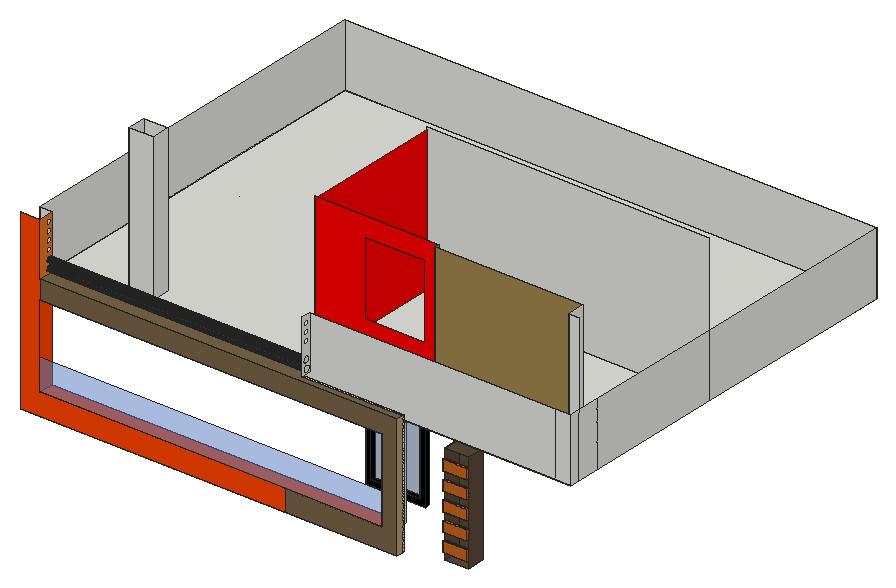
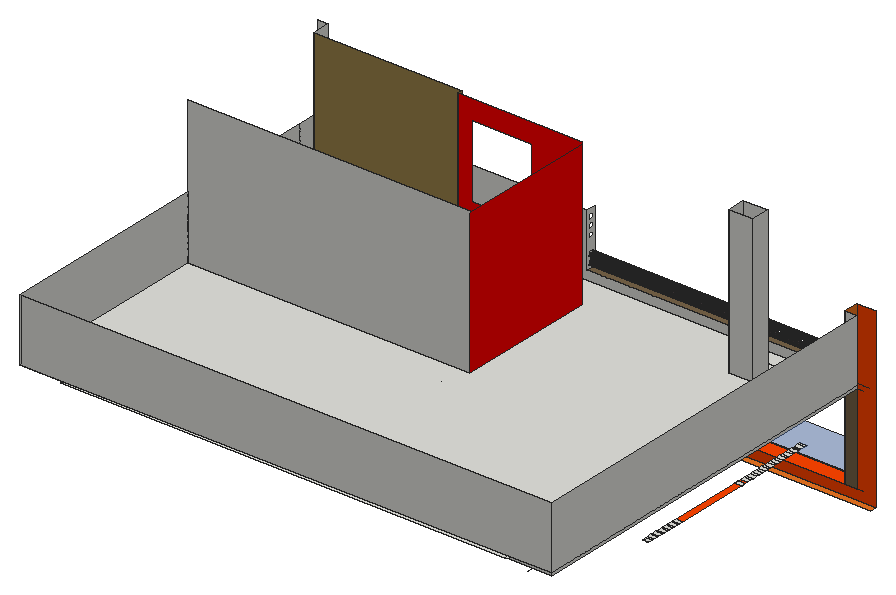
# SketchUp Ruby script. Lengths in inches.
U = 1.inch
M = Sketchup.active_model
def pt(a) = Geom::Point3d.new(a.map { |v| v * U })
def face(e, loops, mat)
  f = e.add_face(loops[0].map { |a| pt(a) })
  loops[1..].each { |l| e.add_face(l.map { |a| pt(a) }).erase! }
  f.material = f.back_material = mat if mat
  f
end
# faces: each face lists its corners as indices into pts; further lists are holes
def faces(e, pts, list, mat = nil) = list.each { |f| face(e, (f[0].is_a?(Array) ? f : [f]).map { |l| l.map { |i| pts[i] } }, mat) }
# xy, xz, yz: faces in a plane at the given z, y or x. An outline is a flat list of corners, or four numbers for a rectangle; further outlines are holes
def ring(l) = l.size == 4 ? [[l[0], l[1]], [l[2], l[1]], [l[2], l[3]], [l[0], l[3]]] : l.each_slice(2).to_a
def flat(e, list, mat, &to3) = list.each { |f| face(e, (f[0].is_a?(Array) ? f : [f]).map { |l| ring(l).map { |u, v| to3.(u, v) } }, mat) }
def xy(e, z, list, mat = nil) = flat(e, list, mat) { |x, y| [x, y, z] }
def xz(e, y, list, mat = nil) = flat(e, list, mat) { |x, z| [x, y, z] }
def yz(e, x, list, mat = nil) = flat(e, list, mat) { |y, z| [x, y, z] }
def lines(e, pts, list) = list.each { |a, b| e.add_line(pt(pts[a]), pt(pts[b])) }
# prism: a flat outline (further loops are holes) pulled along v
def prism(e, loops, v, mat = nil)
  f = face(e, loops, mat); d = Geom::Vector3d.new(v.map { |x| x * U })
  f.pushpull(f.normal.samedirection?(d) ? d.length : -d.length)
end
def box(e, o, s, mat = nil) = prism(e, [[o, [o[0] + s[0], o[1], o[2]], [o[0] + s[0], o[1] + s[1], o[2]], [o[0], o[1] + s[1], o[2]]]], [0, 0, s[2]], mat)
def at(x, y, z, deg = 0) = Geom::Transformation.translation(pt([x, y, z])) * Geom::Transformation.rotation(ORIGIN, Z_AXIS, deg.degrees)
def axes(o, x, y, z) = Geom::Transformation.new([*x, 0, *y, 0, *z, 0, *pt(o).to_a, 1])
def part(name) = M.definitions.add(name)
# library, detail: a bought-in or finely detailed component or shape, given as its bounding box
def library(name, o, s) = part(name).tap { |d| box(d.entities, o, s) }
def detail(e, o, s) = box(e.add_group.entities, o, s)
def put(e, d, t, mat = nil) = e.add_instance(d, t).tap { |i| i.material = mat if mat }
def group(e, t, mat = nil) = e.add_group.tap { |g| g.transformation = t; g.material = mat if mat }.entities
root = M.entities
M.materials.add("[0020_Red]").color = [255, 0, 0]
M.materials.add("[0024_OrangeRed]").color = [255, 69, 0]
M.materials.add("[0036_BurlyWood]1").color = [119, 99, 72]
M.materials.add("[0036_BurlyWood]2").color = [181, 150, 110]
M.materials.add("[0036_BurlyWood]3").color = [89, 73, 54]
M.materials.add("[0036_BurlyWood]5").color = [122, 101, 74]
M.materials.add("[0041_Chocolate]").color = [234, 117, 33]
M.materials.add("[0041_Chocolate]2").color = [198, 99, 28]
M.materials.add("[0137_Black]").color = [0, 0, 0]
M.materials.add("[Asphalt New]").color = [67, 60, 62]
M.materials.add("[Brick Rough Tan]").color = [158, 133, 77]
M.materials.add("[Translucent Glass Blue]").color = [51, 76, 122]
M.materials["[Translucent Glass Blue]"].alpha = 0.5
M.materials.add("[Translucent Glass Blue]1").color = [100, 149, 237]
M.materials["[Translucent Glass Blue]1"].alpha = 0.5
M.materials.add("[Wood Floor]").color = [155, 105, 61]
xy(root,214.625,[[0,236.25,504.125,245.125]],"[0041_Chocolate]")
xy(root,226.86,[[561.28,245.125,593.09,268.0625]],"[0036_BurlyWood]3")
xy(root,228.95,[[398.32,315.9375,478.64,321.9375]],"[0137_Black]")
xy(root,235.22,[[230.26,515.4375,307.58,521.4375]],"[0137_Black]")
xy(root,236.21,[[405.59,315.9375,438.48,321.9375],[447.89,315.9375,471.37,321.9375]],"[0137_Black]")
xy(root,236.74,[[561.28,242.125,593.09,245.125]],"[0041_Chocolate]2")
xy(root,241.22,[[236.26,515.4375,268.92,521.4375],[275.71,515.4375,301.58,521.4375]],"[0137_Black]")
xy(root,243,[[25.71,236.25,484.29,257.25]],"[0024_OrangeRed]")
xy(root,250.24,[[561.28,242.125,593.09,245.125]],"[0041_Chocolate]2")
xy(root,261.24,[[561.28,242.125,593.09,245.125]],"[0041_Chocolate]2")
xy(root,274.74,[[561.28,242.125,593.09,245.125]],"[0041_Chocolate]2")
xy(root,285.74,[[561.28,242.125,593.09,245.125]],"[0041_Chocolate]2")
xy(root,299.24,[[561.28,242.125,593.09,245.125]],"[0041_Chocolate]2")
xy(root,310.24,[[561.28,242.125,593.09,245.125]],"[0041_Chocolate]2")
xy(root,317.78,[[236.26,515.4375,268.92,521.4375],[275.71,515.4375,301.58,521.4375]],"[0137_Black]")
xy(root,323.74,[[561.28,242.125,593.09,245.125]],"[0041_Chocolate]2")
xy(root,323.78,[[230.26,515.4375,307.58,521.4375]],"[0137_Black]")
xy(root,326.0625,[[109.24,515.4375,148.77,521.4375],[155.35,515.4375,188.31,521.4375]],"[0137_Black]")
xy(root,330.81,[[405.59,315.9375,438.48,321.9375],[447.89,315.9375,471.37,321.9375]],"[0137_Black]")
xy(root,334.375,[[348.4375,372.41,351.4375,446.78]])
xy(root,334.74,[[561.28,242.125,593.09,245.125]],"[0041_Chocolate]2")
xy(root,335.17,[[100.13,515.4375,197.41,521.4375]])
xy(root,338.07,[[398.32,315.9375,478.64,321.9375]],"[0137_Black]")
xy(root,339.56,[[0,352.64,9,355.7],[0,355.7,9,361.9],[0,361.9,9,365.65],[0,365.65,9,365.7],[0,365.7,9,371.9],
  [0,371.9,9,375.7],[0,375.7,9,381.9],[0,381.9,9,385.7],[0,385.7,9,391.9],[0,391.9,9,395.7],
  [0,395.7,9,401.9],[0,401.9,9,405.7],[0,405.7,9,411.9],[0,411.9,9,415.7],[0,415.7,9,421.9],
  [0,421.9,9,425.7],[0,425.7,9,431.9],[0,431.9,9,435.7],[0,435.7,9,441.9],[0,441.9,9,445.7],
  [0,445.7,9,451.9],[0,559.26,9,565.46],[0,565.46,9,567.7],[0,567.7,9,573.9],[0,573.9,9,576.14],
  [0,576.14,9,582.34],[0,582.34,9,584.57],[0,584.57,9,590.78],[0,590.78,9,593.01],[0,593.01,9,599.21],
  [0,599.21,9,601.45],[0,601.45,9,607.65],[0,607.65,9,609.89],[0,609.89,9,616.09],[0,616.09,9,616.14]])
xy(root,339.56,[[0,451.9,9,559.26]],"[0024_OrangeRed]")
xy(root,339.69,[[0,455.7,9,461.9]])
xy(root,345.77,[[348.4375,361.01,354.4375,458.18]],"[Wood Floor]")
xy(root,348.24,[[561.28,242.125,593.09,245.125]],"[0041_Chocolate]2")
xy(root,354.29,[[25.71,236.25,484.29,257.25]],"[0036_BurlyWood]1")
xy(root,360.8,[[561.28,245.125,593.09,268.0625]],"[0036_BurlyWood]3")
xy(root,363,[[354.4375,321.9375,354.4375,521.4375,360.4375,521.4375,360.4375,327.9375,665.75,327.9375,665.75,321.9375],[665.75,321.9375,698.375,521.4375],[360.4375,327.9375,665.75,521.4375],[65.25,521.4375,354.4375,527.4375],[354.4375,521.4375,360.4375,527.4375],
  [360.4375,521.4375,665.75,527.4375],[65.25,527.4375,71.25,767.8125],[71.25,527.4375,665.75,767.8125]])
xy(root,363,[[9,257.25,9,767.8125,65.25,767.8125,65.25,521.4375,354.4375,521.4375,354.4375,321.9375,498.8125,321.9375,498.8125,257.25]],"[0036_BurlyWood]5")
xy(root,366,[[[9,257.25,720.125,257.25,720.125,270.98,706.26,270.98,706.26,294.98,507.58,294.98,507.58,300.98,342.3125,300.98,342.3125,488.35,720.125,488.35,720.125,767.8125,9,767.8125],[99.47,277.08,132.15,318.33]],[706.26,270.98,720.125,270.98,720.125,300.98,507.58,300.98,507.58,294.98,706.26,294.98],[99.47,277.08,132.15,293.9],[99.47,293.9,132.15,297.46],[99.47,297.46,132.15,318.33],
  [342.3125,300.98,720.125,488.35]])
xy(root,378.625,[[369.99,245.125,504.125,248.25]])
xy(root,378.625,[[25.71,236.25,504.125,236.25,504.125,245.125,369.99,245.125,369.99,257.25,25.71,257.25]],"[0036_BurlyWood]1")
xz(root,236.25,[[0,214.625,353.27,214.625,353.27,243,25.71,243,25.71,450,0,450]],"[0024_OrangeRed]")
xz(root,236.25,[[353.27,214.625,504.125,214.625,504.125,378.625,25.71,378.625,25.71,354.29,484.29,354.29,484.29,243,353.27,243]],"[0036_BurlyWood]1")
xz(root,236.25,[[25.71,243,484.29,285.4]],"[Translucent Glass Blue]1")
xz(root,242.125,[[561.28,236.74,593.09,250.24],[561.28,261.24,593.09,274.74],[561.28,285.74,593.09,299.24],[561.28,310.24,593.09,323.74],[561.28,334.74,593.09,348.24]],"[0041_Chocolate]2")
xz(root,245.125,[[561.28,236.74,593.09,250.24],[561.28,261.24,593.09,274.74],[561.28,285.74,593.09,299.24],[561.28,310.24,593.09,323.74],[561.28,334.74,593.09,348.24]])
xz(root,248.25,[[498.8125,243,504.125,363]])
xz(root,257.25,[[9,366,9,450,25.71,450,25.71,378.625,369.99,378.625,369.99,450,698.375,450,698.375,366],[698.375,366,720.125,450]])
xz(root,257.25,[[9,243,9,363,498.8125,363,498.8125,243,484.29,243,484.29,354.29,25.71,354.29,25.71,243]],"[0036_BurlyWood]1")
xz(root,268.0625,[[561.28,226.86,593.09,360.8]],"[0036_BurlyWood]3")
xz(root,270.98,[[706.26,366,720.125,561.0625]])
xz(root,293.9,[[99.47,366,132.15,561.0625]])
xz(root,294.98,[[507.58,366,706.26,561.0625]],"[Brick Rough Tan]")
xz(root,300.98,[[[342.3125,366,507.58,561.0625],[408.85,437.16,489.23,535.66]]],"[0020_Red]")
xz(root,315.9375,[[[398.32,228.95,478.64,338.07],[405.59,236.21,438.48,330.81],[447.89,236.21,471.37,330.81]]],"[0137_Black]")
xz(root,318.33,[[99.47,366,132.15,561.0625]])
xz(root,321.9375,[[405.59,236.21,438.48,330.81],[447.89,236.21,471.37,330.81]],"[Translucent Glass Blue]")
xz(root,488.35,[[342.3125,366,720.125,561.0625]])
xz(root,515.4375,[[[230.26,235.22,307.58,323.78],[236.26,241.22,268.92,317.78],[275.71,241.22,301.58,317.78]]],"[0137_Black]")
xz(root,521.4375,[[236.26,241.22,268.92,317.78],[275.71,241.22,301.58,317.78]],"[Translucent Glass Blue]")
xz(root,767.8125,[[9,363,65.25,366],[9,366,720.125,450]])
yz(root,0,[[455.7,339.56,461.9,339.69]])
yz(root,9,[[455.7,339.56,461.9,339.69],[257.25,363,767.8125,366],[257.25,366,767.8125,450]])
yz(root,25.71,[[236.25,243,257.25,354.29]],"[0024_OrangeRed]")
yz(root,25.71,[[[236.25,378.625,257.25,450],[251.48,382.01,250.54,382.14,249.67,382.5,248.92,383.07,248.34,383.82,247.98,384.7,247.86,385.64,247.98,386.58,248.34,387.45,248.92,388.2,249.67,388.78,250.54,389.14,251.48,389.26,252.42,389.14,253.3,388.78,254.05,388.2,254.62,387.45,254.98,386.58,255.11,385.64,254.98,384.7,254.62,383.82,254.05,383.07,253.3,382.5,252.42,382.14],[251.48,392.95,250.54,393.07,249.67,393.44,248.92,394.01,248.34,394.76,247.98,395.64,247.86,396.57,247.98,397.51,248.34,398.39,248.92,399.14,249.67,399.71,250.54,400.08,251.48,400.2,252.42,400.08,253.3,399.71,254.05,399.14,254.62,398.39,254.98,397.51,255.11,396.57,254.98,395.64,254.62,394.76,254.05,394.01,253.3,393.44,252.42,393.07],[251.48,403.89,250.54,404.01,249.67,404.37,248.92,404.95,248.34,405.7,247.98,406.57,247.86,407.51,247.98,408.45,248.34,409.32,248.92,410.08,249.67,410.65,250.54,411.01,251.48,411.14,252.42,411.01,253.3,410.65,254.05,410.08,254.62,409.32,254.98,408.45,255.11,407.51,254.98,406.57,254.62,405.7,254.05,404.95,253.3,404.37,252.42,404.01],[251.48,414.82,250.54,414.95,249.67,415.31,248.92,415.89,248.34,416.64,247.98,417.51,247.86,418.45,247.98,419.39,248.34,420.26,248.92,421.01,249.67,421.59,250.54,421.95,251.48,422.07,252.42,421.95,253.3,421.59,254.05,421.01,254.62,420.26,254.98,419.39,255.11,418.45,254.98,417.51,254.62,416.64,254.05,415.89,253.3,415.31,252.42,414.95],[251.48,425.76,250.54,425.89,249.67,426.25,248.92,426.82,248.34,427.57,247.98,428.45,247.86,429.39,247.98,430.33,248.34,431.2,248.92,431.95,249.67,432.53,250.54,432.89,251.48,433.01,252.42,432.89,253.3,432.53,254.05,431.95,254.62,431.2,254.98,430.33,255.11,429.39,254.98,428.45,254.62,427.57,254.05,426.82,253.3,426.25,252.42,425.89],[251.48,436.7,250.54,436.82,249.67,437.19,248.92,437.76,248.34,438.51,247.98,439.39,247.86,440.32,247.98,441.26,248.34,442.14,248.92,442.89,249.67,443.46,250.54,443.83,251.48,443.95,252.42,443.83,253.3,443.46,254.05,442.89,254.62,442.14,254.98,441.26,255.11,440.32,254.98,439.39,254.62,438.51,254.05,437.76,253.3,437.19,252.42,436.82]]],"[0041_Chocolate]")
yz(root,99.47,[[293.9,366,318.33,561.0625]])
yz(root,132.15,[[293.9,366,318.33,561.0625]])
yz(root,230.26,[[515.4375,235.22,521.4375,323.78]],"[0137_Black]")
yz(root,236.26,[[515.4375,241.22,521.4375,317.78]],"[0137_Black]")
yz(root,268.92,[[515.4375,241.22,521.4375,317.78]],"[0137_Black]")
yz(root,275.71,[[515.4375,241.22,521.4375,317.78]],"[0137_Black]")
yz(root,301.58,[[515.4375,241.22,521.4375,317.78]],"[0137_Black]")
yz(root,307.58,[[515.4375,235.22,521.4375,323.78]],"[0137_Black]")
yz(root,342.3125,[[300.98,366,488.35,557.75]],"[0020_Red]")
yz(root,348.4375,[[427.62,258.41,424.34,258.68,421.23,259.79,418.52,261.66,416.39,264.17,414.98,267.15,414.39,270.4,414.66,273.68,415.76,276.78,417.64,279.49,420.15,281.63,423.13,283.04,426.37,283.63,429.66,283.36,432.76,282.25,435.47,280.38,437.6,277.87,439.02,274.89,439.61,271.65,439.34,268.36,438.23,265.26,436.36,262.55,433.84,260.41,430.86,259]],"[Wood Floor]")
yz(root,369.99,[[[245.125,378.625,257.25,450],[251.48,392.95,252.42,393.07,253.3,393.44,254.05,394.01,254.62,394.76,254.98,395.64,255.11,396.57,254.98,397.51,254.62,398.39,254.05,399.14,253.3,399.71,252.42,400.08,251.48,400.2,250.54,400.08,249.67,399.71,248.92,399.14,248.34,398.39,248.25,398.16,247.98,397.51,247.86,396.57,247.98,395.64,248.25,394.99,248.34,394.76,248.92,394.01,249.67,393.44,250.54,393.07],[251.48,414.82,252.42,414.95,253.3,415.31,254.05,415.89,254.62,416.64,254.98,417.51,255.11,418.45,254.98,419.39,254.62,420.26,254.05,421.01,253.3,421.59,252.42,421.95,251.48,422.07,250.54,421.95,249.67,421.59,248.92,421.01,248.34,420.26,248.25,420.04,247.98,419.39,247.86,418.45,247.98,417.51,248.25,416.86,248.34,416.64,248.92,415.89,249.67,415.31,250.54,414.95],[251.48,436.7,252.42,436.82,253.3,437.19,254.05,437.76,254.62,438.51,254.98,439.39,255.11,440.32,254.98,441.26,254.62,442.14,254.05,442.89,253.3,443.46,252.42,443.83,251.48,443.95,250.54,443.83,249.67,443.46,248.92,442.89,248.34,442.14,248.25,441.91,247.98,441.26,247.86,440.32,247.98,439.39,248.25,438.74,248.34,438.51,248.92,437.76,249.67,437.19,250.54,436.82],[251.48,425.76,252.42,425.89,253.3,426.25,254.05,426.82,254.62,427.57,254.98,428.45,255.11,429.39,254.98,430.33,254.62,431.2,254.05,431.95,253.3,432.53,252.42,432.89,251.48,433.01,250.54,432.89,249.67,432.53,248.92,431.95,248.34,431.2,248.25,430.97,247.98,430.33,247.86,429.39,247.98,428.45,248.25,427.8,248.34,427.57,248.92,426.82,249.67,426.25,250.54,425.89]],[251.48,392.95,252.42,393.07,253.3,393.44,254.05,394.01,254.62,394.76,254.98,395.64,255.11,396.57,254.98,397.51,254.62,398.39,254.05,399.14,253.3,399.71,252.42,400.08,251.48,400.2,250.54,400.08,249.67,399.71,248.92,399.14,248.34,398.39,248.25,398.16,248.25,394.99,248.34,394.76,248.92,394.01,249.67,393.44,250.54,393.07],[248.25,394.99,247.98,395.64,247.86,396.57,247.98,397.51,248.25,398.16]])
yz(root,371.08,[[251.48,382.01,252.42,382.14,253.3,382.5,254.05,383.07,254.62,383.82,254.98,384.7,255.11,385.64,254.98,386.58,254.62,387.45,254.05,388.2,253.3,388.78,252.42,389.14,251.48,389.26,250.54,389.14,249.67,388.78,248.92,388.2,248.34,387.45,247.98,386.58,247.86,385.64,247.98,384.7,248.34,383.82,248.92,383.07,249.67,382.5,250.54,382.14]])
yz(root,398.32,[[315.9375,228.95,321.9375,338.07]],"[0137_Black]")
yz(root,405.59,[[315.9375,236.21,321.9375,330.81]],"[0137_Black]")
yz(root,438.48,[[315.9375,236.21,321.9375,330.81]],"[0137_Black]")
yz(root,447.89,[[315.9375,236.21,321.9375,330.81]],"[0137_Black]")
yz(root,471.37,[[315.9375,236.21,321.9375,330.81]],"[0137_Black]")
yz(root,478.64,[[315.9375,228.95,321.9375,338.07]],"[0137_Black]")
yz(root,484.29,[[236.25,243,257.25,354.29]],"[0036_BurlyWood]1")
yz(root,498.8125,[[248.25,243,257.25,363]])
yz(root,504.125,[[245.125,214.625,248.25,243],[245.125,243,248.25,363],[245.125,363,248.25,378.625]])
yz(root,504.125,[[236.25,214.625,245.125,378.625]],"[0036_BurlyWood]2")
yz(root,507.58,[[294.98,366,300.98,561.0625]],"[Brick Rough Tan]")
yz(root,561.28,[[245.125,226.86,268.0625,360.8]],"[0036_BurlyWood]3")
yz(root,561.28,[[242.125,236.74,245.125,250.24],[242.125,261.24,245.125,274.74],[242.125,285.74,245.125,299.24],[242.125,310.24,245.125,323.74],[242.125,334.74,245.125,348.24]],"[0041_Chocolate]2")
yz(root,593.09,[[245.125,226.86,268.0625,360.8]],"[0036_BurlyWood]3")
yz(root,593.09,[[242.125,236.74,245.125,250.24],[242.125,261.24,245.125,274.74],[242.125,285.74,245.125,299.24],[242.125,310.24,245.125,323.74],[242.125,334.74,245.125,348.24]],"[0041_Chocolate]2")
yz(root,706.26,[[270.98,366,294.98,561.0625]])
yz(root,720.125,[[257.25,366,270.98,450],[270.98,366,300.98,450],[300.98,366,488.35,450],[488.35,366,767.8125,450]])
p = [[351.4375,427.62,258.41],[351.4375,424.34,258.68],[348.4375,424.34,258.68],[348.4375,427.62,258.41],[351.4375,430.86,259],[348.4375,430.86,259],
  [351.4375,421.23,259.79],[348.4375,421.23,259.79],[351.4375,433.84,260.41],[348.4375,433.84,260.41],[351.4375,418.52,261.66],[348.4375,418.52,261.66],
  [351.4375,436.36,262.55],[348.4375,436.36,262.55],[351.4375,416.39,264.17],[348.4375,416.39,264.17],[351.4375,438.23,265.26],[348.4375,438.23,265.26],
  [351.4375,414.98,267.15],[348.4375,414.98,267.15],[351.4375,439.34,268.36],[348.4375,439.34,268.36],[351.4375,414.39,270.4],[348.4375,414.39,270.4],
  [351.4375,439.61,271.65],[348.4375,439.61,271.65],[351.4375,414.66,273.68],[348.4375,414.66,273.68],[351.4375,439.02,274.89],[348.4375,439.02,274.89],
  [351.4375,415.76,276.78],[348.4375,415.76,276.78],[351.4375,437.6,277.87],[348.4375,437.6,277.87],[351.4375,417.64,279.49],[348.4375,417.64,279.49],
  [351.4375,435.47,280.38],[348.4375,435.47,280.38],[351.4375,420.15,281.63],[348.4375,420.15,281.63],[351.4375,432.76,282.25],[348.4375,432.76,282.25],
  [351.4375,423.13,283.04],[348.4375,423.13,283.04],[351.4375,429.66,283.36],[348.4375,429.66,283.36],[351.4375,426.37,283.63],[348.4375,426.37,283.63],
  [25.71,250.54,382.14],[25.71,251.48,382.01],[371.08,251.48,382.01],[371.08,250.54,382.14],[25.71,252.42,382.14],[371.08,252.42,382.14],
  [25.71,249.67,382.5],[371.08,249.67,382.5],[25.71,253.3,382.5],[371.08,253.3,382.5],[25.71,248.92,383.07],[371.08,248.92,383.07],
  [25.71,254.05,383.07],[371.08,254.05,383.07],[25.71,248.34,383.82],[371.08,248.34,383.82],[25.71,254.62,383.82],[371.08,254.62,383.82],
  [25.71,247.98,384.7],[371.08,247.98,384.7],[25.71,254.98,384.7],[371.08,254.98,384.7],[25.71,247.86,385.64],[371.08,247.86,385.64],
  [25.71,255.11,385.64],[371.08,255.11,385.64],[25.71,247.98,386.58],[371.08,247.98,386.58],[25.71,254.98,386.58],[371.08,254.98,386.58],
  [25.71,248.34,387.45],[371.08,248.34,387.45],[25.71,254.62,387.45],[371.08,254.62,387.45],[25.71,248.92,388.2],[371.08,248.92,388.2],
  [25.71,254.05,388.2],[371.08,254.05,388.2],[25.71,249.67,388.78],[371.08,249.67,388.78],[25.71,253.3,388.78],[371.08,253.3,388.78],
  [25.71,250.54,389.14],[371.08,250.54,389.14],[25.71,252.42,389.14],[371.08,252.42,389.14],[25.71,251.48,389.26],[371.08,251.48,389.26],
  [25.71,250.54,393.07],[25.71,251.48,392.95],[369.99,251.48,392.95],[369.99,250.54,393.07],[25.71,252.42,393.07],[369.99,252.42,393.07],
  [25.71,249.67,393.44],[369.99,249.67,393.44],[25.71,253.3,393.44],[369.99,253.3,393.44],[25.71,248.92,394.01],[369.99,248.92,394.01],
  [25.71,254.05,394.01],[369.99,254.05,394.01],[25.71,248.34,394.76],[369.99,248.34,394.76],[25.71,254.62,394.76],[369.99,254.62,394.76],
  [25.71,247.98,395.64],[369.99,248.25,394.99],[369.99,247.98,395.64],[25.71,254.98,395.64],[369.99,254.98,395.64],[25.71,247.86,396.57],
  [369.99,247.86,396.57],[25.71,255.11,396.57],[369.99,255.11,396.57],[25.71,247.98,397.51],[369.99,247.98,397.51],[25.71,254.98,397.51],
  [369.99,254.98,397.51],[25.71,248.34,398.39],[369.99,248.25,398.16],[369.99,248.34,398.39],[25.71,254.62,398.39],[369.99,254.62,398.39],
  [25.71,248.92,399.14],[369.99,248.92,399.14],[25.71,254.05,399.14],[369.99,254.05,399.14],[0,365.7,340.69],[9,365.7,340.69],
  [665.75,321.9375,363],[665.75,321.9375,366],[354.4375,521.4375,363],[354.4375,521.4375,366],[65.25,521.4375,363],[65.25,521.4375,366],
  [354.4375,321.9375,363],[354.4375,321.9375,366],[498.8125,248.25,363],[0,248.25,363],[9,257.25,243],[0,257.25,243],
  [9,257.25,363],[0,257.25,363],[34.5625,767.8125,363],[34.5625,776.8125,363]]
faces(root,p,[[0,1,2,3],[4,0,3,5],[1,6,7,2],[8,4,5,9],[6,10,11,7],[12,8,9,13],[10,14,15,11],[16,12,13,17],
  [14,18,19,15],[20,16,17,21],[18,22,23,19],[24,20,21,25],[22,26,27,23],[28,24,25,29],[26,30,31,27],[32,28,29,33],
  [30,34,35,31],[36,32,33,37],[34,38,39,35],[40,36,37,41],[38,42,43,39],[44,40,41,45],[42,46,47,43],[46,44,45,47]],"[Wood Floor]")
faces(root,p,[[48,49,50,51],[49,52,53,50],[54,48,51,55],[52,56,57,53],[58,54,55,59],[56,60,61,57],[62,58,59,63],[60,64,65,61],
  [66,62,63,67],[64,68,69,65],[70,66,67,71],[68,72,73,69],[74,70,71,75],[72,76,77,73],[78,74,75,79],[76,80,81,77],
  [82,78,79,83],[80,84,85,81],[86,82,83,87],[84,88,89,85],[90,86,87,91],[88,92,93,89],[94,90,91,95],[92,94,95,93],
  [96,97,98,99],[97,100,101,98],[102,96,99,103],[100,104,105,101],[106,102,103,107],[104,108,109,105],[110,106,107,111],[108,112,113,109],
  [114,110,111,115,116],[112,117,118,113],[119,114,116,120],[117,121,122,118],[123,119,120,124],[121,125,126,122],[127,123,124,128,129],[125,130,131,126],
  [132,127,129,133],[130,134,135,131]],"[Asphalt New]")
lines(root,p,[[136,137],[138,139],[140,141],[142,143],[144,145],[146,147],[148,149],[150,151],[152,153]])
